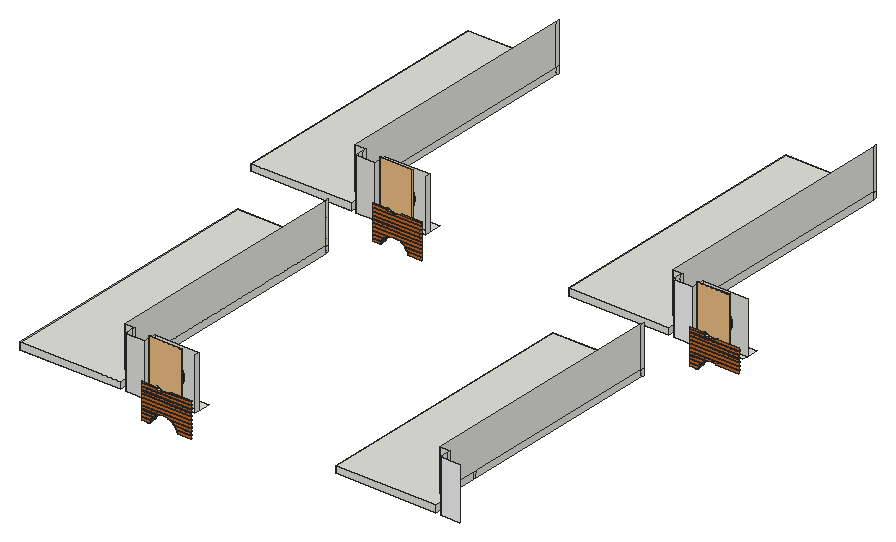
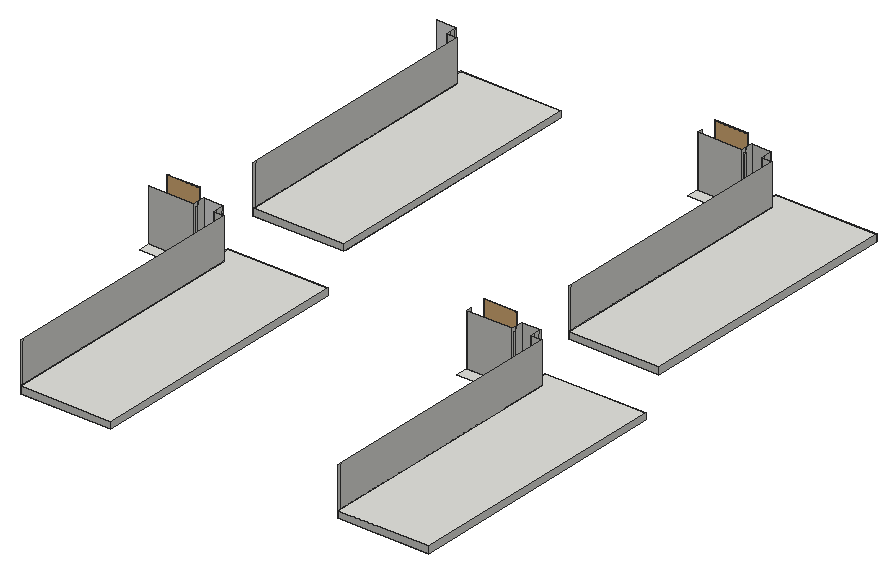
# SketchUp Ruby script. Lengths in inches.
U = 1.inch
M = Sketchup.active_model
def pt(a) = Geom::Point3d.new(a.map { |v| v * U })
def face(e, loops, mat)
  f = e.add_face(loops[0].map { |a| pt(a) })
  loops[1..].each { |l| e.add_face(l.map { |a| pt(a) }).erase! }
  f.material = f.back_material = mat if mat
  f
end
# faces: each face lists its corners as indices into pts; further lists are holes
def faces(e, pts, list, mat = nil) = list.each { |f| face(e, (f[0].is_a?(Array) ? f : [f]).map { |l| l.map { |i| pts[i] } }, mat) }
# xy, xz, yz: faces in a plane at the given z, y or x. An outline is a flat list of corners, or four numbers for a rectangle; further outlines are holes
def ring(l) = l.size == 4 ? [[l[0], l[1]], [l[2], l[1]], [l[2], l[3]], [l[0], l[3]]] : l.each_slice(2).to_a
def flat(e, list, mat, &to3) = list.each { |f| face(e, (f[0].is_a?(Array) ? f : [f]).map { |l| ring(l).map { |u, v| to3.(u, v) } }, mat) }
def xy(e, z, list, mat = nil) = flat(e, list, mat) { |x, y| [x, y, z] }
def xz(e, y, list, mat = nil) = flat(e, list, mat) { |x, z| [x, y, z] }
def yz(e, x, list, mat = nil) = flat(e, list, mat) { |y, z| [x, y, z] }
def lines(e, pts, list) = list.each { |a, b| e.add_line(pt(pts[a]), pt(pts[b])) }
# prism: a flat outline (further loops are holes) pulled along v
def prism(e, loops, v, mat = nil)
  f = face(e, loops, mat); d = Geom::Vector3d.new(v.map { |x| x * U })
  f.pushpull(f.normal.samedirection?(d) ? d.length : -d.length)
end
def box(e, o, s, mat = nil) = prism(e, [[o, [o[0] + s[0], o[1], o[2]], [o[0] + s[0], o[1] + s[1], o[2]], [o[0], o[1] + s[1], o[2]]]], [0, 0, s[2]], mat)
def at(x, y, z, deg = 0) = Geom::Transformation.translation(pt([x, y, z])) * Geom::Transformation.rotation(ORIGIN, Z_AXIS, deg.degrees)
def axes(o, x, y, z) = Geom::Transformation.new([*x, 0, *y, 0, *z, 0, *pt(o).to_a, 1])
def part(name) = M.definitions.add(name)
# library, detail: a bought-in or finely detailed component or shape, given as its bounding box
def library(name, o, s) = part(name).tap { |d| box(d.entities, o, s) }
def detail(e, o, s) = box(e.add_group.entities, o, s)
def put(e, d, t, mat = nil) = e.add_instance(d, t).tap { |i| i.material = mat if mat }
def group(e, t, mat = nil) = e.add_group.tap { |g| g.transformation = t; g.material = mat if mat }.entities
root = M.entities
M.materials.add("[0041_Chocolate]").color = [210, 105, 30]
M.materials.add("[0129_WhiteSmoke]").color = [245, 245, 245]
M.materials.add("[Color M06]").color = [84, 84, 84]
M.materials.add("[Color M08]").color = [30, 30, 30]
c1 = library("1",[3.97,34.78,0],[101.43,33.99,0.79])
xy(root,260.375,[[897.211,280.466,913.525,281.466],[971.242,280.466,998.644,281.466],[820.523,971.36,836.838,972.36],[894.555,971.36,921.956,972.36],[1476.023,971.36,1492.338,972.36]],"[0041_Chocolate]")
xy(root,265.329,[[897.211,280.466,915.395,281.466],[969.373,280.466,998.644,281.466],[820.523,971.36,838.707,972.36],[892.685,971.36,921.956,972.36],[1476.023,971.36,1494.207,972.36]],"[0041_Chocolate]")
xy(root,267.4375,[[897.211,280.466,916.268,281.466],[968.5,280.466,998.644,281.466],[820.523,971.36,839.58,972.36],[891.812,971.36,921.956,972.36],[1476.023,971.36,1495.08,972.36]],"[0041_Chocolate]")
xy(root,272.392,[[897.211,280.466,919.798,281.466],[964.97,280.466,998.644,281.466],[820.523,971.36,843.11,972.36],[888.282,971.36,921.956,972.36],[1476.023,971.36,1498.61,972.36]],"[0041_Chocolate]")
xy(root,274.5,[[897.211,280.466,921.482,281.466],[963.286,280.466,998.644,281.466],[820.523,971.36,844.795,972.36],[886.598,971.36,921.956,972.36],[1476.023,971.36,1500.295,972.36]],"[0041_Chocolate]")
xy(root,279.454,[[897.211,280.466,928.321,281.466],[956.446,280.466,998.644,281.466],[820.523,971.36,851.634,972.36],[879.759,971.36,921.956,972.36],[1476.023,971.36,1507.134,972.36]],"[0041_Chocolate]")
xy(root,281.5625,[[897.211,280.466,933.411,281.466],[951.357,280.466,998.644,281.466],[820.523,971.36,856.723,972.36],[874.669,971.36,921.956,972.36],[1476.023,971.36,1512.223,972.36]],"[0041_Chocolate]")
xy(root,286.517,[[897.211,280.466,998.644,281.466],[820.523,971.36,921.956,972.36],[1476.023,971.36,1577.456,972.36]],"[0041_Chocolate]")
xy(root,288.625,[[897.211,280.466,998.644,281.466],[820.523,971.36,921.956,972.36],[1476.023,971.36,1577.456,972.36]],"[0041_Chocolate]")
xy(root,293.579,[[897.211,280.466,998.644,281.466],[820.523,971.36,921.956,972.36],[1476.023,971.36,1577.456,972.36]],"[0041_Chocolate]")
xy(root,295.6875,[[897.211,280.466,998.644,281.466],[820.523,971.36,921.956,972.36],[1476.023,971.36,1577.456,972.36]],"[0041_Chocolate]")
xy(root,295.724,[[857.243,287.951,897.211,337.5625],[897.211,302.0625,990.023,312.8125],[897.211,312.8125,990.023,337.5625],[780.555,978.845,820.523,1028.457],[1436.055,978.845,1476.023,1028.457],
  [820.523,992.957,913.336,1003.707],[1476.023,992.957,1568.836,1003.707],[820.523,1003.707,913.336,1028.457],[1476.023,1003.707,1568.836,1028.457]])
xy(root,300.642,[[897.211,280.466,998.644,281.466],[820.523,971.36,921.956,972.36],[1476.023,971.36,1577.456,972.36]],"[0041_Chocolate]")
xy(root,302.75,[[897.211,280.466,998.644,281.466],[820.523,971.36,921.956,972.36],[1476.023,971.36,1577.456,972.36]],"[0041_Chocolate]")
xy(root,304.253,[[648.897,277.25,648.897,830.913,657.44,830.913,657.44,341.872,657.689,338.079,658.43,334.351,659.652,330.752,661.333,327.342,662.672,325.339,663.445,324.182,664.225,323.293,665.952,321.324,668.809,318.818,671.97,316.706,675.379,315.025,678.979,313.803,682.707,313.061,686.5,312.8125,856.378,312.8125,856.378,277.25],[1299.397,277.25,1299.397,830.913,1307.94,830.913,1307.94,341.872,1308.189,338.079,1308.93,334.351,1310.152,330.752,1311.833,327.342,1313.172,325.339,1313.945,324.182,1314.725,323.293,1316.452,321.324,1319.309,318.818,1322.47,316.706,1325.879,315.025,1329.479,313.803,1333.207,313.061,1337,312.8125,1506.878,312.8125,1506.878,277.25],[686.5,312.8125,836.003,312.8125,836.003,325.339,692.245,325.339,688.587,325.579,684.993,326.294,681.522,327.472,678.235,329.093,675.187,331.129,672.432,333.546,670.015,336.301,667.979,339.349,666.358,342.636,665.179,346.107,664.464,349.702,664.225,353.359,664.225,323.293,665.952,321.324,668.809,318.818,671.97,316.706,675.379,315.025,678.979,313.803,682.707,313.061],[1337,312.8125,1486.503,312.8125,1486.503,325.339,1342.745,325.339,1339.087,325.579,1335.493,326.294,1332.022,327.472,1328.735,329.093,1325.687,331.129,1322.932,333.546,1320.515,336.301,1318.479,339.349,1316.858,342.636,1315.679,346.107,1314.964,349.702,1314.725,353.359,1314.725,323.293,1316.452,321.324,1319.309,318.818,1322.47,316.706,1325.879,315.025,1329.479,313.803,1333.207,313.061],[664.225,323.293,664.225,830.913,657.44,830.913,657.44,341.872,657.689,338.079,658.43,334.351,659.652,330.752,661.333,327.342,662.672,325.339,663.445,324.182],
  [1314.725,323.293,1314.725,830.913,1307.94,830.913,1307.94,341.872,1308.189,338.079,1308.93,334.351,1310.152,330.752,1311.833,327.342,1313.172,325.339,1313.945,324.182],[692.245,325.339,688.587,325.579,684.993,326.294,681.522,327.472,678.235,329.093,675.187,331.129,672.432,333.546,670.015,336.301,667.979,339.349,666.358,342.636,665.179,346.107,664.464,349.702,664.225,353.359,664.225,830.913,836.003,830.913,836.003,325.339],[1342.745,325.339,1339.087,325.579,1335.493,326.294,1332.022,327.472,1328.735,329.093,1325.687,331.129,1322.932,333.546,1320.515,336.301,1318.479,339.349,1316.858,342.636,1315.679,346.107,1314.964,349.702,1314.725,353.359,1314.725,830.913,1486.503,830.913,1486.503,325.339],[648.897,830.913,836.003,838.144],[1299.397,830.913,1486.503,838.144],
  [572.209,968.144,572.209,1521.808,580.753,1521.808,580.753,1032.767,581.001,1028.973,581.743,1025.245,582.965,1021.646,584.646,1018.237,585.985,1016.233,586.758,1015.076,587.537,1014.187,589.264,1012.218,592.122,1009.712,595.282,1007.6,598.692,1005.919,602.291,1004.697,606.019,1003.955,609.8125,1003.707,779.69,1003.707,779.69,968.144],[1227.709,968.144,1227.709,1521.808,1236.253,1521.808,1236.253,1032.767,1236.501,1028.973,1237.243,1025.245,1238.465,1021.646,1240.146,1018.237,1241.485,1016.233,1242.258,1015.076,1243.037,1014.187,1244.764,1012.218,1247.622,1009.712,1250.782,1007.6,1254.192,1005.919,1257.791,1004.697,1261.519,1003.955,1265.3125,1003.707,1435.19,1003.707,1435.19,968.144],[609.8125,1003.707,759.315,1003.707,759.315,1016.233,615.557,1016.233,611.9,1016.473,608.305,1017.188,604.834,1018.366,601.547,1019.987,598.5,1022.023,595.744,1024.44,593.327,1027.196,591.291,1030.243,589.67,1033.53,588.492,1037.001,587.777,1040.596,587.537,1044.253,587.537,1014.187,589.264,1012.218,592.122,1009.712,595.282,1007.6,598.692,1005.919,602.291,1004.697,606.019,1003.955],[1265.3125,1003.707,1414.815,1003.707,1414.815,1016.233,1271.057,1016.233,1267.4,1016.473,1263.805,1017.188,1260.334,1018.366,1257.047,1019.987,1254,1022.023,1251.244,1024.44,1248.827,1027.196,1246.791,1030.243,1245.17,1033.53,1243.992,1037.001,1243.277,1040.596,1243.037,1044.253,1243.037,1014.187,1244.764,1012.218,1247.622,1009.712,1250.782,1007.6,1254.192,1005.919,1257.791,1004.697,1261.519,1003.955],[587.537,1014.187,587.537,1521.808,580.753,1521.808,580.753,1032.767,581.001,1028.973,581.743,1025.245,582.965,1021.646,584.646,1018.237,585.985,1016.233,586.758,1015.076],
  [1243.037,1014.187,1243.037,1521.808,1236.253,1521.808,1236.253,1032.767,1236.501,1028.973,1237.243,1025.245,1238.465,1021.646,1240.146,1018.237,1241.485,1016.233,1242.258,1015.076],[615.557,1016.233,611.9,1016.473,608.305,1017.188,604.834,1018.366,601.547,1019.987,598.5,1022.023,595.744,1024.44,593.327,1027.196,591.291,1030.243,589.67,1033.53,588.492,1037.001,587.777,1040.596,587.537,1044.253,587.537,1521.808,759.315,1521.808,759.315,1016.233],[1271.057,1016.233,1267.4,1016.473,1263.805,1017.188,1260.334,1018.366,1257.047,1019.987,1254,1022.023,1251.244,1024.44,1248.827,1027.196,1246.791,1030.243,1245.17,1033.53,1243.992,1037.001,1243.277,1040.596,1243.037,1044.253,1243.037,1521.808,1414.815,1521.808,1414.815,1016.233],[572.209,1521.808,759.315,1529.038],[1227.709,1521.808,1414.815,1529.038]])
xy(root,307.704,[[897.211,280.466,998.644,281.466],[820.523,971.36,921.956,972.36],[1476.023,971.36,1577.456,972.36]],"[0041_Chocolate]")
xy(root,309.8125,[[897.211,280.466,998.644,281.466],[820.523,971.36,921.956,972.36],[1476.023,971.36,1577.456,972.36]],"[0041_Chocolate]")
xy(root,314.767,[[897.211,280.466,998.644,281.466],[820.523,971.36,921.956,972.36],[1476.023,971.36,1577.456,972.36]],"[0041_Chocolate]")
xy(root,316.875,[[897.211,280.466,998.644,281.466],[820.523,971.36,921.956,972.36],[1476.023,971.36,1577.456,972.36]],"[0041_Chocolate]")
xy(root,318.066,[[648.897,277.25,856.378,277.25,856.378,312.8125,836.003,312.8125,836.003,838.144,648.897,838.144],[1299.397,277.25,1506.878,277.25,1506.878,312.8125,1486.503,312.8125,1486.503,838.144,1299.397,838.144],[572.209,968.144,779.69,968.144,779.69,1003.707,759.315,1003.707,759.315,1529.038,572.209,1529.038],[1227.709,968.144,1435.19,968.144,1435.19,1003.707,1414.815,1003.707,1414.815,1529.038,1227.709,1529.038]])
xy(root,321.829,[[897.211,280.466,998.644,281.466],[820.523,971.36,921.956,972.36],[1476.023,971.36,1577.456,972.36]],"[0041_Chocolate]")
xy(root,323.9375,[[897.211,280.466,998.644,281.466],[820.523,971.36,921.956,972.36],[1476.023,971.36,1577.456,972.36]],"[0041_Chocolate]")
xy(root,328.892,[[897.211,280.466,927.356,281.466],[953.875,280.466,998.644,281.466],[820.523,971.36,850.669,972.36],[877.1875,971.36,921.956,972.36],[1476.023,971.36,1506.169,972.36]],"[0041_Chocolate]")
xz(root,277.25,[[648.897,304.253,856.378,318.066],[1299.397,304.253,1506.878,318.066]])
xz(root,280.466,[[897.211,260.375,913.525,260.375,913.611,261.022,915.395,265.329,897.211,265.329],[971.242,260.375,998.644,260.375,998.644,265.329,969.373,265.329,971.157,261.022],[897.211,267.4375,916.268,267.4375,916.586,268.207,919.798,272.392,897.211,272.392],[968.5,267.4375,998.644,267.4375,998.644,272.392,964.97,272.392,968.181,268.207],[897.211,274.5,921.482,274.5,927.49,279.11,928.321,279.454,897.211,279.454],
  [963.286,274.5,998.644,274.5,998.644,279.454,956.446,279.454,957.278,279.11],[897.211,281.5625,933.411,281.5625,934.674,282.086,942.384,283.101,950.094,282.086,951.357,281.5625,998.644,281.5625,998.644,286.517,897.211,286.517],[897.211,288.625,998.644,293.579],[897.211,295.6875,998.644,300.642],[897.211,302.75,998.644,307.704],
  [897.211,309.8125,998.644,314.767],[897.211,316.875,998.644,321.829],[897.211,323.9375,998.644,323.9375,998.644,328.892,953.875,328.892,952.631,328.172,944.723,326.049,936.536,326.045,928.626,328.16,927.356,328.892,897.211,328.892]],"[0041_Chocolate]")
xz(root,281.466,[[897.211,265.329,915.395,265.329,916.268,267.4375,897.211,267.4375],[969.373,265.329,998.644,265.329,998.644,267.4375,968.5,267.4375],[897.211,272.392,919.798,272.392,921.32,274.376,921.482,274.5,897.211,274.5],[964.97,272.392,998.644,272.392,998.644,274.5,963.286,274.5,963.447,274.376],[897.211,279.454,928.321,279.454,933.411,281.5625,897.211,281.5625],
  [956.446,279.454,998.644,279.454,998.644,281.5625,951.357,281.5625],[897.211,286.517,998.644,288.625],[897.211,293.579,998.644,295.6875],[897.211,300.642,998.644,302.75],[897.211,307.704,998.644,309.8125],
  [897.211,314.767,998.644,316.875],[897.211,321.829,998.644,323.9375],[897.211,328.892,927.356,328.892,923.7,331,897.211,331],[953.875,328.892,998.644,328.892,998.644,331,957.522,331]],"[0041_Chocolate]")
xz(root,287.951,[[857.243,295.724,897.211,402.635]])
xz(root,287.951,[[1507.743,295.724,1547.711,402.635]],"[0129_WhiteSmoke]")
xz(root,295.653,[[936.536,326.045,944.723,326.049,952.631,328.172,953.875,328.892,957.522,331,959.719,332.27,963.399,335.954,965.505,338.0625,968.362,343.017,969.578,345.125,969.595,345.155,970.912,350.079,971.475,352.1875,971.71,353.065,971.708,357.142,971.707,359.25,971.706,361.252,970.913,364.204,970.347,366.3125,969.582,369.16,968.364,371.267,967.254,373.1875,965.485,376.248,963.589,378.142,961.666,380.0625,959.692,382.034,954.52,385.017,952.599,386.124,949.557,386.9375,944.69,388.239,936.502,388.234,931.673,386.9375,928.595,386.111,926.702,385.017,921.507,382.014,919.558,380.0625,917.639,378.142,915.721,376.221,913.971,373.1875,912.864,371.267,911.631,369.128,910.878,366.3125,910.314,364.204,909.516,361.219,909.517,359.25,909.518,357.142,909.52,353.031,909.747,352.1875,910.313,350.079,911.643,345.125,911.644,345.124,912.862,343.017,915.726,338.0625,915.741,338.036,917.825,335.954,921.534,332.249,923.7,331,927.356,328.892,928.626,328.16]],"[Color M08]")
xz(root,312.8125,[[897.211,295.724,990.023,402.635],[836.003,304.253,856.378,318.066],[856.378,304.253,857.243,309.691],[1486.503,304.253,1506.878,318.066],[1506.878,304.253,1507.743,309.691],
  [856.378,309.691,857.243,309.691,857.243,402.635,836.003,402.635,836.003,318.066,856.378,318.066],[1506.878,309.691,1507.743,309.691,1507.743,402.635,1486.503,402.635,1486.503,318.066,1506.878,318.066]])
xz(root,838.144,[[648.897,304.253,836.003,318.066],[1299.397,304.253,1486.503,318.066]])
xz(root,968.144,[[572.209,304.253,779.69,318.066],[1227.709,304.253,1435.19,318.066]])
xz(root,971.36,[[820.523,260.375,836.838,260.375,836.923,261.022,838.707,265.329,820.523,265.329],[894.555,260.375,921.956,260.375,921.956,265.329,892.685,265.329,894.469,261.022],[1476.023,260.375,1492.338,260.375,1492.423,261.022,1494.207,265.329,1476.023,265.329],[820.523,267.4375,839.58,267.4375,839.899,268.207,843.11,272.392,820.523,272.392],[891.812,267.4375,921.956,267.4375,921.956,272.392,888.282,272.392,891.494,268.207],
  [1476.023,267.4375,1495.08,267.4375,1495.399,268.207,1498.61,272.392,1476.023,272.392],[820.523,274.5,844.795,274.5,850.802,279.11,851.634,279.454,820.523,279.454],[886.598,274.5,921.956,274.5,921.956,279.454,879.759,279.454,880.59,279.11],[1476.023,274.5,1500.295,274.5,1506.302,279.11,1507.134,279.454,1476.023,279.454],[820.523,281.5625,856.723,281.5625,857.987,282.086,865.696,283.101,873.406,282.086,874.669,281.5625,921.956,281.5625,921.956,286.517,820.523,286.517],
  [1476.023,281.5625,1512.223,281.5625,1513.487,282.086,1521.196,283.101,1528.906,282.086,1530.169,281.5625,1577.456,281.5625,1577.456,286.517,1476.023,286.517],[820.523,288.625,921.956,293.579],[1476.023,288.625,1577.456,293.579],[820.523,295.6875,921.956,300.642],[1476.023,295.6875,1577.456,300.642],
  [820.523,302.75,921.956,307.704],[1476.023,302.75,1577.456,307.704],[820.523,309.8125,921.956,314.767],[1476.023,309.8125,1577.456,314.767],[820.523,316.875,921.956,321.829],
  [1476.023,316.875,1577.456,321.829],[820.523,323.9375,921.956,323.9375,921.956,328.892,877.1875,328.892,875.943,328.172,868.036,326.049,859.848,326.045,851.939,328.16,850.669,328.892,820.523,328.892],[1476.023,323.9375,1577.456,323.9375,1577.456,328.892,1532.6875,328.892,1531.443,328.172,1523.536,326.049,1515.348,326.045,1507.439,328.16,1506.169,328.892,1476.023,328.892]],"[0041_Chocolate]")
xz(root,972.36,[[820.523,265.329,838.707,265.329,839.58,267.4375,820.523,267.4375],[892.685,265.329,921.956,265.329,921.956,267.4375,891.812,267.4375],[1476.023,265.329,1494.207,265.329,1495.08,267.4375,1476.023,267.4375],[820.523,272.392,843.11,272.392,844.633,274.376,844.795,274.5,820.523,274.5],[888.282,272.392,921.956,272.392,921.956,274.5,886.598,274.5,886.76,274.376],
  [1476.023,272.392,1498.61,272.392,1500.133,274.376,1500.295,274.5,1476.023,274.5],[820.523,279.454,851.634,279.454,856.723,281.5625,820.523,281.5625],[879.759,279.454,921.956,279.454,921.956,281.5625,874.669,281.5625],[1476.023,279.454,1507.134,279.454,1512.223,281.5625,1476.023,281.5625],[820.523,286.517,921.956,288.625],
  [1476.023,286.517,1577.456,288.625],[820.523,293.579,921.956,295.6875],[1476.023,293.579,1577.456,295.6875],[820.523,300.642,921.956,302.75],[1476.023,300.642,1577.456,302.75],
  [820.523,307.704,921.956,309.8125],[1476.023,307.704,1577.456,309.8125],[820.523,314.767,921.956,316.875],[1476.023,314.767,1577.456,316.875],[820.523,321.829,921.956,323.9375],
  [1476.023,321.829,1577.456,323.9375],[820.523,328.892,850.669,328.892,847.013,331,820.523,331],[877.1875,328.892,921.956,328.892,921.956,331,880.835,331],[1476.023,328.892,1506.169,328.892,1502.513,331,1476.023,331]],"[0041_Chocolate]")
xz(root,978.845,[[780.555,295.724,820.523,402.635]])
xz(root,978.845,[[1436.055,295.724,1476.023,402.635]],"[0129_WhiteSmoke]")
xz(root,986.548,[[859.848,326.045,868.036,326.049,875.943,328.172,877.1875,328.892,880.835,331,883.032,332.27,886.712,335.954,888.818,338.0625,891.675,343.017,892.89,345.125,892.908,345.155,894.224,350.079,894.788,352.1875,895.022,353.065,895.02,357.142,895.019,359.25,895.018,361.252,894.225,364.204,893.659,366.3125,892.895,369.16,891.677,371.267,890.566,373.1875,888.797,376.248,886.901,378.142,884.978,380.0625,883.005,382.034,877.832,385.017,875.912,386.124,872.87,386.9375,868.002,388.239,859.815,388.234,854.985,386.9375,851.908,386.111,850.015,385.017,844.819,382.014,842.87,380.0625,840.952,378.142,839.033,376.221,837.284,373.1875,836.176,371.267,834.943,369.128,834.19,366.3125,833.627,364.204,832.828,361.219,832.829,359.25,832.831,357.142,832.833,353.031,833.059,352.1875,833.625,350.079,834.956,345.125,834.956,345.124,836.174,343.017,839.038,338.0625,839.054,338.036,841.137,335.954,844.846,332.249,847.013,331,850.669,328.892,851.939,328.16],[1515.348,326.045,1523.536,326.049,1531.443,328.172,1532.6875,328.892,1536.335,331,1538.532,332.27,1542.212,335.954,1544.318,338.0625,1547.175,343.017,1548.39,345.125,1548.408,345.155,1549.724,350.079,1550.288,352.1875,1550.522,353.065,1550.52,357.142,1550.519,359.25,1550.518,361.252,1549.725,364.204,1549.159,366.3125,1548.395,369.16,1547.177,371.267,1546.066,373.1875,1544.297,376.248,1542.401,378.142,1540.478,380.0625,1538.505,382.034,1533.332,385.017,1531.412,386.124,1528.37,386.9375,1523.502,388.239,1515.315,388.234,1510.485,386.9375,1507.408,386.111,1505.515,385.017,1500.319,382.014,1498.37,380.0625,1496.452,378.142,1494.533,376.221,1492.784,373.1875,1491.676,371.267,1490.443,369.128,1489.69,366.3125,1489.127,364.204,1488.328,361.219,1488.329,359.25,1488.331,357.142,1488.333,353.031,1488.559,352.1875,1489.125,350.079,1490.456,345.125,1490.456,345.124,1491.674,343.017,1494.538,338.0625,1494.554,338.036,1496.637,335.954,1500.346,332.249,1502.513,331,1506.169,328.892,1507.439,328.16]],"[Color M08]")
xz(root,1003.707,[[820.523,295.724,913.336,402.635],[1476.023,295.724,1568.836,402.635],[759.315,304.253,779.69,318.066],[779.69,304.253,780.555,309.691],[1414.815,304.253,1435.19,318.066],
  [1435.19,304.253,1436.055,309.691],[779.69,309.691,780.555,309.691,780.555,402.635,759.315,402.635,759.315,318.066,779.69,318.066],[1435.19,309.691,1436.055,309.691,1436.055,402.635,1414.815,402.635,1414.815,318.066,1435.19,318.066]])
xz(root,1529.038,[[572.209,304.253,759.315,318.066],[1227.709,304.253,1414.815,318.066]])
yz(root,572.209,[[968.144,304.253,1529.038,318.066]])
yz(root,648.897,[[277.25,304.253,838.144,318.066]])
yz(root,759.315,[[1003.707,304.253,1088.752,318.066],[1088.752,304.253,1097.276,318.066],[1097.276,304.253,1521.808,318.066],[1521.808,304.253,1529.038,318.066],[1003.707,318.066,1521.808,402.635],
  [1521.808,318.066,1529.038,402.635]])
yz(root,779.69,[[968.144,304.253,1003.707,318.066]])
yz(root,780.555,[[978.845,295.724,983.345,304.253],[983.345,295.724,996.476,304.253],[996.476,295.724,1003.707,304.253],[978.845,304.253,983.345,309.691],[983.345,304.253,996.476,309.691],
  [996.476,304.253,1003.707,309.691],[978.845,309.691,983.345,402.635],[983.345,309.691,996.476,402.635],[996.476,309.691,1003.707,402.635]])
yz(root,820.523,[[978.845,295.724,993.351,295.724,993.351,395.26,991.226,395.26,991.226,402.635,978.845,402.635],[993.351,295.724,996.476,395.26],[1001.163,295.724,1003.707,295.724,1003.707,402.635,996.476,402.635,996.476,395.26,1001.163,395.26],[996.476,295.724,1001.163,395.26]])
yz(root,836.003,[[312.8125,304.253,397.858,318.066],[397.858,304.253,406.382,318.066],[406.382,304.253,830.913,318.066],[830.913,304.253,838.144,318.066],[312.8125,318.066,830.913,402.635],
  [830.913,318.066,838.144,402.635]])
yz(root,856.378,[[277.25,304.253,312.8125,318.066]])
yz(root,857.243,[[287.951,295.724,292.451,304.253],[292.451,295.724,305.582,304.253],[305.582,295.724,312.8125,304.253],[287.951,304.253,292.451,309.691],[292.451,304.253,305.582,309.691],
  [305.582,304.253,312.8125,309.691],[287.951,309.691,292.451,402.635],[292.451,309.691,305.582,402.635],[305.582,309.691,312.8125,402.635]])
yz(root,897.211,[[287.951,295.724,302.457,295.724,302.457,395.26,300.332,395.26,300.332,402.635,287.951,402.635],[302.457,295.724,305.582,395.26],[305.582,295.724,310.269,395.26],[310.269,295.724,312.8125,295.724,312.8125,402.635,305.582,402.635,305.582,395.26,310.269,395.26]])
yz(root,913.336,[[993.351,295.724,1003.707,402.635]])
yz(root,990.023,[[302.457,295.724,312.8125,402.635]])
yz(root,1227.709,[[968.144,304.253,1529.038,318.066]])
yz(root,1299.397,[[277.25,304.253,838.144,318.066]])
yz(root,1414.815,[[1003.707,304.253,1088.752,318.066],[1088.752,304.253,1097.276,318.066],[1097.276,304.253,1521.808,318.066],[1521.808,304.253,1529.038,318.066],[1003.707,318.066,1521.808,402.635],
  [1521.808,318.066,1529.038,402.635]])
yz(root,1435.19,[[968.144,304.253,1003.707,318.066]])
yz(root,1436.055,[[978.845,295.724,983.345,304.253],[983.345,295.724,996.476,304.253],[996.476,295.724,1003.707,304.253],[978.845,304.253,983.345,309.691],[983.345,304.253,996.476,309.691],
  [996.476,304.253,1003.707,309.691],[978.845,309.691,983.345,402.635],[983.345,309.691,996.476,402.635],[996.476,309.691,1003.707,402.635]])
yz(root,1476.023,[[978.845,295.724,993.351,295.724,993.351,395.26,991.226,395.26,991.226,402.635,978.845,402.635],[993.351,295.724,996.476,395.26],[1001.163,295.724,1003.707,295.724,1003.707,402.635,996.476,402.635,996.476,395.26,1001.163,395.26],[996.476,295.724,1001.163,395.26]])
yz(root,1486.503,[[312.8125,304.253,397.858,318.066],[397.858,304.253,406.382,318.066],[406.382,304.253,830.913,318.066],[830.913,304.253,838.144,318.066],[312.8125,318.066,830.913,402.635],
  [830.913,318.066,838.144,402.635]])
yz(root,1506.878,[[277.25,304.253,312.8125,318.066]])
yz(root,1507.743,[[287.951,295.724,292.451,304.253],[292.451,295.724,305.582,304.253],[305.582,295.724,312.8125,304.253],[287.951,304.253,292.451,309.691],[292.451,304.253,305.582,309.691],
  [305.582,304.253,312.8125,309.691],[287.951,309.691,292.451,402.635],[292.451,309.691,305.582,402.635],[305.582,309.691,312.8125,402.635]])
p = [[913.611,295.653,261.022],[913.611,280.466,261.022],[913.525,280.466,260.375],[913.525,281.466,260.375],[913.525,295.653,260.375],[971.242,295.653,260.375],
  [971.242,281.466,260.375],[971.242,280.466,260.375],[971.157,280.466,261.022],[971.157,295.653,261.022],[836.923,986.548,261.022],[836.923,971.36,261.022],
  [836.838,971.36,260.375],[836.838,972.36,260.375],[836.838,986.548,260.375],[894.555,986.548,260.375],[894.555,972.36,260.375],[894.555,971.36,260.375],
  [894.469,971.36,261.022],[894.469,986.548,261.022],[1492.423,986.548,261.022],[1492.423,971.36,261.022],[1492.338,971.36,260.375],[1492.338,972.36,260.375],
  [1492.338,986.548,260.375],[915.395,295.653,265.329],[915.395,281.466,265.329],[915.395,280.466,265.329],[969.373,280.466,265.329],[969.373,281.466,265.329],
  [969.373,295.653,265.329],[838.707,986.548,265.329],[838.707,972.36,265.329],[838.707,971.36,265.329],[892.685,971.36,265.329],[892.685,972.36,265.329],
  [892.685,986.548,265.329],[1494.207,986.548,265.329],[1494.207,972.36,265.329],[1494.207,971.36,265.329],[916.268,281.466,267.4375],[916.268,295.653,267.4375],
  [968.5,281.466,267.4375],[968.5,295.653,267.4375],[839.58,972.36,267.4375],[839.58,986.548,267.4375],[891.812,972.36,267.4375],[891.812,986.548,267.4375],
  [1495.08,972.36,267.4375],[1495.08,986.548,267.4375],[916.586,295.653,268.207],[916.586,280.466,268.207],[916.268,280.466,267.4375],[968.5,280.466,267.4375],
  [968.181,280.466,268.207],[968.181,295.653,268.207],[839.899,986.548,268.207],[839.899,971.36,268.207],[839.58,971.36,267.4375],[891.812,971.36,267.4375],
  [891.494,971.36,268.207],[891.494,986.548,268.207],[1495.399,986.548,268.207],[1495.399,971.36,268.207],[1495.08,971.36,267.4375],[919.798,295.653,272.392],
  [919.798,281.466,272.392],[919.798,280.466,272.392],[964.97,280.466,272.392],[964.97,281.466,272.392],[964.97,295.653,272.392],[843.11,986.548,272.392],
  [843.11,972.36,272.392],[843.11,971.36,272.392],[888.282,971.36,272.392],[888.282,972.36,272.392],[888.282,986.548,272.392],[1498.61,986.548,272.392],
  [1498.61,972.36,272.392],[1498.61,971.36,272.392],[921.32,281.466,274.376],[921.32,295.653,274.376],[963.447,281.466,274.376],[963.447,295.653,274.376],
  [844.633,972.36,274.376],[844.633,986.548,274.376],[886.76,972.36,274.376],[886.76,986.548,274.376],[1500.133,972.36,274.376],[1500.133,986.548,274.376],
  [921.482,281.466,274.5],[921.482,295.653,274.5],[963.286,281.466,274.5],[963.286,295.653,274.5],[844.795,972.36,274.5],[844.795,986.548,274.5],
  [886.598,972.36,274.5],[886.598,986.548,274.5],[1500.295,972.36,274.5],[1500.295,986.548,274.5],[927.49,295.653,279.11],[927.49,280.466,279.11],
  [921.482,280.466,274.5],[963.286,280.466,274.5],[957.278,280.466,279.11],[957.278,295.653,279.11],[850.802,986.548,279.11],[850.802,971.36,279.11],
  [844.795,971.36,274.5],[886.598,971.36,274.5],[880.59,971.36,279.11],[880.59,986.548,279.11],[1506.302,986.548,279.11],[1506.302,971.36,279.11],
  [1500.295,971.36,274.5],[928.321,295.653,279.454],[928.321,281.466,279.454],[928.321,280.466,279.454],[956.446,280.466,279.454],[956.446,281.466,279.454],
  [956.446,295.653,279.454],[851.634,986.548,279.454],[851.634,972.36,279.454],[851.634,971.36,279.454],[879.759,971.36,279.454],[879.759,972.36,279.454],
  [879.759,986.548,279.454],[1507.134,986.548,279.454],[1507.134,972.36,279.454],[1507.134,971.36,279.454],[933.411,281.466,281.5625],[933.411,295.653,281.5625],
  [951.357,281.466,281.5625],[951.357,295.653,281.5625],[856.723,972.36,281.5625],[856.723,986.548,281.5625],[874.669,972.36,281.5625],[874.669,986.548,281.5625],
  [1512.223,972.36,281.5625],[1512.223,986.548,281.5625],[934.674,295.653,282.086],[934.674,280.466,282.086],[933.411,280.466,281.5625],[951.357,280.466,281.5625],
  [950.094,280.466,282.086],[950.094,295.653,282.086],[857.987,986.548,282.086],[857.987,971.36,282.086],[856.723,971.36,281.5625],[874.669,971.36,281.5625],
  [873.406,971.36,282.086],[873.406,986.548,282.086],[1513.487,986.548,282.086],[1513.487,971.36,282.086],[1512.223,971.36,281.5625],[942.384,295.653,283.101],
  [942.384,280.466,283.101],[865.696,986.548,283.101],[865.696,971.36,283.101],[1521.196,986.548,283.101],[1521.196,971.36,283.101],[1528.906,986.548,282.086],
  [1528.906,971.36,282.086],[928.626,295.653,328.16],[928.626,280.466,328.16],[936.536,280.466,326.045],[936.536,295.653,326.045],[944.723,280.466,326.049],
  [944.723,295.653,326.049],[952.631,280.466,328.172],[952.631,295.653,328.172],[851.939,986.548,328.16],[851.939,971.36,328.16],[859.848,971.36,326.045],
  [859.848,986.548,326.045],[868.036,971.36,326.049],[868.036,986.548,326.049],[875.943,971.36,328.172],[875.943,986.548,328.172],[1507.439,986.548,328.16],
  [1507.439,971.36,328.16],[1515.348,971.36,326.045],[1515.348,986.548,326.045],[1523.536,971.36,326.049],[1523.536,986.548,326.049],[1531.443,971.36,328.172],
  [1531.443,986.548,328.172],[927.356,295.653,328.892],[927.356,281.466,328.892],[927.356,280.466,328.892],[953.875,280.466,328.892],[953.875,281.466,328.892],
  [953.875,295.653,328.892],[850.669,986.548,328.892],[850.669,972.36,328.892],[850.669,971.36,328.892],[877.1875,971.36,328.892],[877.1875,972.36,328.892],
  [877.1875,986.548,328.892],[1506.169,986.548,328.892],[1506.169,972.36,328.892],[1506.169,971.36,328.892],[923.7,281.466,331],[923.7,295.653,331],
  [957.522,281.466,331],[957.522,295.653,331],[847.013,972.36,331],[847.013,986.548,331],[880.835,972.36,331],[880.835,986.548,331],
  [1502.513,972.36,331],[1502.513,986.548,331]]
faces(root,p,[[0,1,2,3,4],[5,6,7,8,9],[10,11,12,13,14],[15,16,17,18,19],[20,21,22,23,24],[25,26,27,1,0],[9,8,28,29,30],[31,32,33,11,10],
  [19,18,34,35,36],[37,38,39,21,20],[40,26,25,41],[29,42,43,30],[44,32,31,45],[35,46,47,36],[48,38,37,49],[50,51,52,40,41],
  [43,42,53,54,55],[56,57,58,44,45],[47,46,59,60,61],[62,63,64,48,49],[65,66,67,51,50],[55,54,68,69,70],[71,72,73,57,56],[61,60,74,75,76],
  [77,78,79,63,62],[80,66,65,81],[69,82,83,70],[84,72,71,85],[75,86,87,76],[88,78,77,89],[90,80,81,91],[82,92,93,83],
  [94,84,85,95],[86,96,97,87],[98,88,89,99],[100,101,102,90,91],[93,92,103,104,105],[106,107,108,94,95],[97,96,109,110,111],[112,113,114,98,99],
  [115,116,117,101,100],[105,104,118,119,120],[121,122,123,107,106],[111,110,124,125,126],[127,128,129,113,112],[130,116,115,131],[119,132,133,120],[134,122,121,135],
  [125,136,137,126],[138,128,127,139],[140,141,142,130,131],[133,132,143,144,145],[146,147,148,134,135],[137,136,149,150,151],[152,153,154,138,139],[155,156,141,140],
  [145,144,156,155],[157,158,147,146],[151,150,158,157],[159,160,153,152],[161,162,160,159]],"[Color M06]")
faces(root,p,[[163,164,165,166],[166,165,167,168],[168,167,169,170],[171,172,173,174],[174,173,175,176],[176,175,177,178],[179,180,181,182],[182,181,183,184],
  [184,183,185,186],[187,188,189,164,163],[170,169,190,191,192],[193,194,195,172,171],[178,177,196,197,198],[199,200,201,180,179],[202,188,187,203],[191,204,205,192],
  [206,194,193,207],[197,208,209,198],[210,200,199,211]])
put(root,c1,axes([968.59,977.04,312.08],[0,0,1],[-2,0,0],[0,-1,0]))
put(root,c1,axes([1045.27,286.15,312.08],[0,0,1],[-2,0,0],[0,-1,0]))
put(root,c1,axes([1624.09,977.04,312.08],[0,0,1],[-2,0,0],[0,-1,0]))
